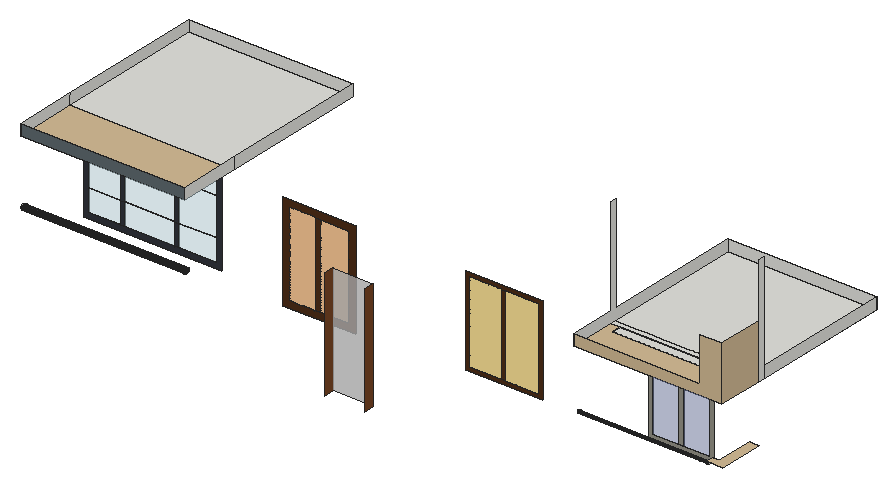
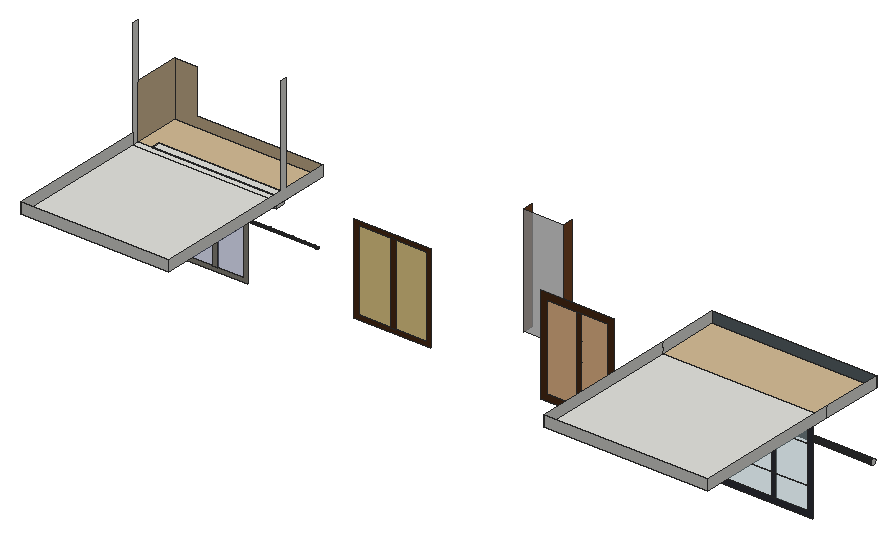
# SketchUp Ruby script. Lengths in inches.
U = 1.inch
M = Sketchup.active_model
def pt(a) = Geom::Point3d.new(a.map { |v| v * U })
def face(e, loops, mat)
  f = e.add_face(loops[0].map { |a| pt(a) })
  loops[1..].each { |l| e.add_face(l.map { |a| pt(a) }).erase! }
  f.material = f.back_material = mat if mat
  f
end
# faces: each face lists its corners as indices into pts; further lists are holes
def faces(e, pts, list, mat = nil) = list.each { |f| face(e, (f[0].is_a?(Array) ? f : [f]).map { |l| l.map { |i| pts[i] } }, mat) }
# xy, xz, yz: faces in a plane at the given z, y or x. An outline is a flat list of corners, or four numbers for a rectangle; further outlines are holes
def ring(l) = l.size == 4 ? [[l[0], l[1]], [l[2], l[1]], [l[2], l[3]], [l[0], l[3]]] : l.each_slice(2).to_a
def flat(e, list, mat, &to3) = list.each { |f| face(e, (f[0].is_a?(Array) ? f : [f]).map { |l| ring(l).map { |u, v| to3.(u, v) } }, mat) }
def xy(e, z, list, mat = nil) = flat(e, list, mat) { |x, y| [x, y, z] }
def xz(e, y, list, mat = nil) = flat(e, list, mat) { |x, z| [x, y, z] }
def yz(e, x, list, mat = nil) = flat(e, list, mat) { |y, z| [x, y, z] }
def lines(e, pts, list) = list.each { |a, b| e.add_line(pt(pts[a]), pt(pts[b])) }
# prism: a flat outline (further loops are holes) pulled along v
def prism(e, loops, v, mat = nil)
  f = face(e, loops, mat); d = Geom::Vector3d.new(v.map { |x| x * U })
  f.pushpull(f.normal.samedirection?(d) ? d.length : -d.length)
end
def box(e, o, s, mat = nil) = prism(e, [[o, [o[0] + s[0], o[1], o[2]], [o[0] + s[0], o[1] + s[1], o[2]], [o[0], o[1] + s[1], o[2]]]], [0, 0, s[2]], mat)
def at(x, y, z, deg = 0) = Geom::Transformation.translation(pt([x, y, z])) * Geom::Transformation.rotation(ORIGIN, Z_AXIS, deg.degrees)
def axes(o, x, y, z) = Geom::Transformation.new([*x, 0, *y, 0, *z, 0, *pt(o).to_a, 1])
def part(name) = M.definitions.add(name)
# library, detail: a bought-in or finely detailed component or shape, given as its bounding box
def library(name, o, s) = part(name).tap { |d| box(d.entities, o, s) }
def detail(e, o, s) = box(e.add_group.entities, o, s)
def put(e, d, t, mat = nil) = e.add_instance(d, t).tap { |i| i.material = mat if mat }
def group(e, t, mat = nil) = e.add_group.tap { |g| g.transformation = t; g.material = mat if mat }.entities
root = M.entities
M.materials.add("[Color C02]").color = [255, 204, 153]
M.materials.add("[Color D02]").color = [255, 229, 153]
M.materials.add("[Formica Beige]").color = [211, 187, 149]
M.materials.add("[Formica Graystone]").color = [149, 146, 135]
M.materials.add("[Formica Laminate Dark]").color = [50, 53, 60]
M.materials.add("[Formica Speckled Grey]").color = [94, 105, 111]
M.materials.add("[Translucent Glass Safety]").color = [204, 235, 244]
M.materials["[Translucent Glass Safety]"].alpha = 0.5
M.materials.add("[Translucent Glass Sky Reflection]").color = [126, 138, 183]
M.materials["[Translucent Glass Sky Reflection]"].alpha = 0.52
M.materials.add("[Translucent Resin Crush Gray]").color = [201, 201, 201]
M.materials["[Translucent Resin Crush Gray]"].alpha = 0.8
M.materials.add("[Wood Floor Light]").color = [204, 176, 127]
M.materials.add("[Wood Veneer 01]").color = [79, 46, 24]
M.materials.add("[Wood Veneer 01]2").color = [120, 70, 37]
xy(root,295.875,[[13.84,125.42,14.27,125.48,14.68,125.65,15.03,125.92,15.3,126.27,15.47,126.67,15.52,127.11,15.47,127.55,15.3,127.95,15.03,128.3,14.68,128.57,14.27,128.74,13.84,128.8,13.4,128.74,12.99,128.57,12.64,128.3,12.375,127.95,12.21,127.55,12.15,127.11,12.21,126.67,12.375,126.27,12.64,125.92,12.99,125.65,13.4,125.48]])
xy(root,296.125,[[101.27,125.42,101.71,125.48,102.12,125.65,102.47,125.92,102.74,126.27,102.9,126.67,102.96,127.11,102.9,127.55,102.74,127.95,102.47,128.3,102.12,128.57,101.71,128.74,101.27,128.8,100.84,128.74,100.43,128.57,100.08,128.3,99.8125,127.95,99.64,127.55,99.59,127.11,99.64,126.67,99.8125,126.27,100.08,125.92,100.43,125.65,100.84,125.48]])
xy(root,296.5,[[133.84,125.42,134.27,125.48,134.68,125.65,135.03,125.92,135.3,126.27,135.47,126.67,135.52,127.11,135.47,127.55,135.3,127.95,135.03,128.3,134.68,128.57,134.27,128.74,133.84,128.8,133.4,128.74,132.99,128.57,132.64,128.3,132.375,127.95,132.21,127.55,132.15,127.11,132.21,126.67,132.375,126.27,132.64,125.92,132.99,125.65,133.4,125.48]])
xy(root,296.625,[[118.77,125.42,119.21,125.48,119.62,125.65,119.97,125.92,120.24,126.27,120.4,126.67,120.46,127.11,120.4,127.55,120.24,127.95,119.97,128.3,119.62,128.57,119.21,128.74,118.77,128.8,118.34,128.74,117.93,128.57,117.58,128.3,117.3125,127.95,117.14,127.55,117.09,127.11,117.14,126.67,117.3125,126.27,117.58,125.92,117.93,125.65,118.34,125.48]])
xy(root,297.375,[[71.27,125.42,71.71,125.48,72.12,125.65,72.47,125.92,72.74,126.27,72.9,126.67,72.96,127.11,72.9,127.55,72.74,127.95,72.47,128.3,72.12,128.57,71.71,128.74,71.27,128.8,70.84,128.74,70.43,128.57,70.08,128.3,69.8125,127.95,69.64,127.55,69.59,127.11,69.64,126.67,69.8125,126.27,70.08,125.92,70.43,125.65,70.84,125.48]])
xy(root,297.49,[[42.4,125.42,42.84,125.48,43.24,125.65,43.59,125.92,43.86,126.27,44.03,126.67,44.09,127.11,44.03,127.55,43.86,127.95,43.59,128.3,43.24,128.57,42.84,128.74,42.4,128.8,41.96,128.74,41.56,128.57,41.21,128.3,40.9375,127.95,40.77,127.55,40.71,127.11,40.77,126.67,40.9375,126.27,41.21,125.92,41.56,125.65,41.96,125.48]])
xy(root,298.1875,[[27.09,125.42,27.52,125.48,27.93,125.65,28.28,125.92,28.55,126.27,28.72,126.67,28.77,127.11,28.72,127.55,28.55,127.95,28.28,128.3,27.93,128.57,27.52,128.74,27.09,128.8,26.65,128.74,26.24,128.57,25.89,128.3,25.625,127.95,25.46,127.55,25.4,127.11,25.46,126.67,25.625,126.27,25.89,125.92,26.24,125.65,26.65,125.48],[55.4,125.42,55.84,125.48,56.24,125.65,56.59,125.92,56.86,126.27,57.03,126.67,57.09,127.11,57.03,127.55,56.86,127.95,56.59,128.3,56.24,128.57,55.84,128.74,55.4,128.8,54.96,128.74,54.56,128.57,54.21,128.3,53.9375,127.95,53.77,127.55,53.71,127.11,53.77,126.67,53.9375,126.27,54.21,125.92,54.56,125.65,54.96,125.48],[149.84,125.42,150.27,125.48,150.68,125.65,151.03,125.92,151.3,126.27,151.47,126.67,151.52,127.11,151.47,127.55,151.3,127.95,151.03,128.3,150.68,128.57,150.27,128.74,149.84,128.8,149.4,128.74,148.99,128.57,148.64,128.3,148.375,127.95,148.21,127.55,148.15,127.11,148.21,126.67,148.375,126.27,148.64,125.92,148.99,125.65,149.4,125.48]])
xy(root,298.84,[[86.21,125.42,86.65,125.48,87.06,125.65,87.41,125.92,87.67,126.27,87.84,126.67,87.9,127.11,87.84,127.55,87.67,127.95,87.41,128.3,87.06,128.57,86.65,128.74,86.21,128.8,85.78,128.74,85.37,128.57,85.02,128.3,84.75,127.95,84.58,127.55,84.52,127.11,84.58,126.67,84.75,126.27,85.02,125.92,85.37,125.65,85.78,125.48],[167.96,125.42,168.4,125.48,168.81,125.65,169.16,125.92,169.42,126.27,169.59,126.67,169.65,127.11,169.59,127.55,169.42,127.95,169.16,128.3,168.81,128.57,168.4,128.74,167.96,128.8,167.53,128.74,167.12,128.57,166.77,128.3,166.5,127.95,166.33,127.55,166.27,127.11,166.33,126.67,166.5,126.27,166.77,125.92,167.12,125.65,167.53,125.48],[183.34,125.42,183.77,125.48,184.18,125.65,184.53,125.92,184.8,126.27,184.97,126.67,185.02,127.11,184.97,127.55,184.8,127.95,184.53,128.3,184.18,128.57,183.77,128.74,183.34,128.8,182.9,128.74,182.49,128.57,182.14,128.3,181.875,127.95,181.71,127.55,181.65,127.11,181.71,126.67,181.875,126.27,182.14,125.92,182.49,125.65,182.9,125.48]])
xy(root,301.75,[[674.41,135.92,674.75,135.96,675.07,136.09,675.34,136.3,675.55,136.57,675.68,136.89,675.72,137.23,675.68,137.57,675.55,137.88,675.34,138.16,675.07,138.36,674.75,138.5,674.41,138.54,674.07,138.5,673.75,138.36,673.48,138.16,673.27,137.88,673.14,137.57,673.1,137.23,673.14,136.89,673.27,136.57,673.48,136.3,673.75,136.09,674.07,135.96]],"[Formica Laminate Dark]")
xy(root,301.8125,[[628.3,136.16,628.61,136.2,628.9,136.32,629.14,136.51,629.33,136.76,629.45,137.04,629.49,137.35,629.45,137.66,629.33,137.94,629.14,138.19,628.9,138.38,628.61,138.5,628.3,138.54,627.99,138.5,627.71,138.38,627.46,138.19,627.27,137.94,627.16,137.66,627.11,137.35,627.16,137.04,627.27,136.76,627.46,136.51,627.71,136.32,627.99,136.2]],"[Formica Laminate Dark]")
xy(root,301.875,[[746.55,136.16,746.86,136.2,747.15,136.32,747.39,136.51,747.58,136.76,747.7,137.04,747.74,137.35,747.7,137.66,747.58,137.94,747.39,138.19,747.15,138.38,746.86,138.5,746.55,138.54,746.24,138.5,745.96,138.38,745.71,138.19,745.52,137.94,745.41,137.66,745.36,137.35,745.41,137.04,745.52,136.76,745.71,136.51,745.96,136.32,746.24,136.2]],"[Formica Laminate Dark]")
xy(root,301.91,[[651.47,136.9,653.64,136.9,653.7,137.04,653.74,137.35,653.7,137.66,653.58,137.94,653.39,138.19,653.15,138.38,652.86,138.5,652.55,138.54,652.24,138.5,651.96,138.38,651.71,138.19,651.52,137.94,651.41,137.66,651.36,137.35,651.41,137.04]])
xy(root,301.91,[[652.55,136.16,652.86,136.2,653.15,136.32,653.39,136.51,653.58,136.76,653.64,136.9,651.47,136.9,651.52,136.76,651.71,136.51,651.96,136.32,652.24,136.2]],"[Formica Laminate Dark]")
xy(root,301.9375,[[701.43,136.16,701.73,136.2,702.02,136.32,702.27,136.51,702.46,136.76,702.57,137.04,702.61,137.35,702.57,137.66,702.46,137.94,702.27,138.19,702.02,138.38,701.73,138.5,701.43,138.54,701.12,138.5,700.83,138.38,700.59,138.19,700.4,137.94,700.28,137.66,700.24,137.35,700.28,137.04,700.4,136.76,700.59,136.51,700.83,136.32,701.12,136.2]],"[Formica Laminate Dark]")
xy(root,302.125,[[684.99,136.16,685.3,136.2,685.58,136.32,685.83,136.51,686.02,136.76,686.14,137.04,686.18,137.35,686.14,137.66,686.02,137.94,685.83,138.19,685.58,138.38,685.3,138.5,684.99,138.54,684.68,138.5,684.4,138.38,684.15,138.19,683.96,137.94,683.84,137.66,683.8,137.35,683.84,137.04,683.96,136.76,684.15,136.51,684.4,136.32,684.68,136.2]],"[Formica Laminate Dark]")
xy(root,302.1875,[[735.74,136.16,736.05,136.2,736.33,136.32,736.58,136.51,736.77,136.76,736.89,137.04,736.93,137.35,736.89,137.66,736.77,137.94,736.58,138.19,736.33,138.38,736.05,138.5,735.74,138.54,735.43,138.5,735.15,138.38,734.9,138.19,734.71,137.94,734.59,137.66,734.55,137.35,734.59,137.04,734.71,136.76,734.9,136.51,735.15,136.32,735.43,136.2]],"[Formica Laminate Dark]")
xy(root,302.22,[[616.26,136.9375,618.47,136.9375,618.51,137.04,618.55,137.35,618.51,137.66,618.39,137.94,618.2,138.19,617.96,138.38,617.67,138.5,617.36,138.54,617.06,138.5,616.77,138.38,616.52,138.19,616.34,137.94,616.22,137.66,616.18,137.35,616.22,137.04]])
xy(root,302.22,[[617.36,136.16,617.67,136.2,617.96,136.32,618.2,136.51,618.39,136.76,618.47,136.9375,616.26,136.9375,616.34,136.76,616.52,136.51,616.77,136.32,617.06,136.2]],"[Formica Laminate Dark]")
xy(root,302.3125,[[640.36,136.16,640.67,136.2,640.96,136.32,641.2,136.51,641.39,136.76,641.51,137.04,641.55,137.35,641.51,137.66,641.39,137.94,641.2,138.19,640.96,138.38,640.67,138.5,640.36,138.54,640.06,138.5,639.77,138.38,639.52,138.19,639.34,137.94,639.22,137.66,639.18,137.35,639.22,137.04,639.34,136.76,639.52,136.51,639.77,136.32,640.06,136.2],[713.18,136.16,713.48,136.2,713.77,136.32,714.02,136.51,714.21,136.76,714.32,137.04,714.36,137.35,714.32,137.66,714.21,137.94,714.02,138.19,713.77,138.38,713.48,138.5,713.18,138.54,712.87,138.5,712.58,138.38,712.34,138.19,712.15,137.94,712.03,137.66,711.99,137.35,712.03,137.04,712.15,136.76,712.34,136.51,712.58,136.32,712.87,136.2]],"[Formica Laminate Dark]")
xy(root,302.375,[[724.8,136.16,725.11,136.2,725.4,136.32,725.64,136.51,725.83,136.76,725.95,137.04,725.99,137.35,725.95,137.66,725.83,137.94,725.64,138.19,725.4,138.38,725.11,138.5,724.8,138.54,724.49,138.5,724.21,138.38,723.96,138.19,723.77,137.94,723.66,137.66,723.61,137.35,723.66,137.04,723.77,136.76,723.96,136.51,724.21,136.32,724.49,136.2]],"[Formica Laminate Dark]")
xy(root,302.51,[[691.18,137.06,693.76,137.06,693.79,137.23,693.74,137.57,693.61,137.88,693.4,138.16,693.13,138.36,692.8125,138.5,692.47,138.54,692.13,138.5,691.82,138.36,691.55,138.16,691.34,137.88,691.21,137.57,691.16,137.23]])
xy(root,302.51,[[692.47,135.92,692.8125,135.96,693.13,136.09,693.4,136.3,693.61,136.57,693.74,136.89,693.76,137.06,691.18,137.06,691.21,136.89,691.34,136.57,691.55,136.3,691.82,136.09,692.13,135.96]],"[Formica Laminate Dark]")
xy(root,302.8125,[[665.36,136.16,665.67,136.2,665.96,136.32,666.2,136.51,666.39,136.76,666.51,137.04,666.55,137.35,666.51,137.66,666.39,137.94,666.2,138.19,665.96,138.38,665.67,138.5,665.36,138.54,665.06,138.5,664.77,138.38,664.52,138.19,664.34,137.94,664.22,137.66,664.18,137.35,664.22,137.04,664.34,136.76,664.52,136.51,664.77,136.32,665.06,136.2]],"[Formica Laminate Dark]")
xy(root,305.625,[[755.9375,133.3,774.15,133.3,774.15,182.57,764,182.57,764,141.82,755.9375,141.82]],"[Formica Beige]")
xy(root,356.625,[[621.3,172.64,641.63,182.57],[738.55,172.64,758.88,182.57]])
xy(root,356.625,[[641.63,172.64,738.55,182.57]],"[Wood Floor Light]")
xy(root,369,[[621.3,172.64,758.88,182.57],[621.3,172.64,758.88,182.57],[611.125,182.57,774.15,189.24],[611.125,189.24,774.15,344.36],[9,191.15,189.57,355.125]])
xy(root,369,[[9,122.79,189.57,191.15],[611.125,131.74,611.125,182.57,621.3,182.57,621.3,172.64,758.88,172.64,758.88,182.57,774.15,182.57,774.15,131.74]],"[Formica Beige]")
xz(root,88.2,[[380.3,262.65,424.94,384.08]],"[Translucent Resin Crush Gray]")
xz(root,122.79,[[9,369,189.57,381]],"[Formica Speckled Grey]")
xz(root,131.74,[[611.125,369,774.15,369,774.15,429,750.32,429,750.32,381,611.125,381]],"[Formica Beige]")
xz(root,172.64,[[621.3,356.625,758.88,369]],"[Wood Floor Light]")
xz(root,174.4375,[[264.12,273.03,292.18,365.2],[298.29,273.03,329.29,365.2]],"[Color C02]")
xz(root,174.4375,[[462.79,277.61,496.49,366.55],[502.51,277.61,537.84,366.55]],"[Color D02]")
xz(root,174.4375,[[[256.64,265.55,336.77,372.68],[264.12,273.03,329.29,365.2]],[292.18,273.03,298.29,365.2],[[458.21,273.03,542.42,371.125],[462.79,277.61,537.84,366.55]],[496.49,277.61,502.51,366.55]],"[Wood Veneer 01]")
xz(root,182.57,[[621.3,356.625,758.88,369]])
xz(root,182.57,[[[653.42,271.33,724.17,352.83],[657.48,275.39,720.12,348.77]],[685.82,275.39,691.11,348.77]],"[Formica Graystone]")
xz(root,182.57,[[657.48,275.39,685.82,348.77],[691.11,275.39,720.12,348.77]],"[Translucent Glass Sky Reflection]")
xz(root,191.15,[[[24.08,264.5,176.08,363],[29.79,270.2,170.375,357.29]],[64.72,270.2,69.58,294.48],[124.16,270.2,129.01,294.48],[64.72,294.48,69.58,336.17],[124.16,294.48,129.01,336.17],
  [64.72,336.17,69.58,357.29],[124.16,336.17,129.01,357.29]],"[Formica Laminate Dark]")
xz(root,191.15,[[29.79,270.2,64.72,294.48],[69.58,270.2,124.16,294.48],[129.01,270.2,170.375,294.48],[29.79,294.48,64.72,336.17],[69.58,294.48,124.16,336.17],
  [129.01,294.48,170.375,336.17],[29.79,336.17,64.72,357.29],[69.58,336.17,124.16,357.29],[129.01,336.17,170.375,357.29]],"[Translucent Glass Safety]")
xz(root,344.36,[[611.125,369,774.15,381]])
xz(root,355.125,[[9,369,189.57,381]])
yz(root,9,[[126.49,294.81,125.8,294.9,125.15,295.17,124.59,295.59,124.17,296.15,123.9,296.8,123.81,297.49,123.9,298.1875,124.17,298.84,124.59,299.39,125.15,299.82,125.8,300.09,126.49,300.18,127.1875,300.09,127.84,299.82,128.39,299.39,128.82,298.84,129.09,298.1875,129.18,297.49,129.09,296.8,128.82,296.15,128.39,295.59,127.84,295.17,127.1875,294.9],[122.79,369,191.15,381],[191.15,369,355.125,381]])
yz(root,189.57,[[122.79,369,191.15,381],[191.15,369,355.125,381]])
yz(root,380.3,[[77.26,262.65,88.2,384.08]],"[Wood Veneer 01]2")
yz(root,424.94,[[77.26,262.65,88.2,384.08]],"[Wood Veneer 01]2")
yz(root,611.125,[[131.74,369,344.36,369,344.36,381,189.24,381,189.24,489,182.57,489,182.57,381,131.74,381]])
yz(root,621.3,[[172.64,356.625,182.57,369]])
yz(root,755.9375,[[138.08,300.72,138.39,300.77,138.68,300.88,138.92,301.07,139.11,301.32,139.23,301.6,139.27,301.91,139.23,302.22,139.11,302.51,138.92,302.75,138.68,302.94,138.39,303.06,138.08,303.1,137.78,303.06,137.49,302.94,137.25,302.75,137.06,302.51,136.9375,302.22,136.9,301.91,136.9375,301.6,137.06,301.32,137.25,301.07,137.49,300.88,137.78,300.77]])
yz(root,758.88,[[172.64,356.625,182.57,369]],"[Formica Beige]")
yz(root,774.15,[[182.57,369,189.24,489],[189.24,369,344.36,381]])
yz(root,774.15,[[131.74,369,182.57,429]],"[Formica Beige]")
p = [[9,125.8,294.9],[9,126.49,294.81],[189.57,126.49,294.81],[189.57,125.8,294.9],[9,127.1875,294.9],[189.57,127.1875,294.9],
  [9,125.15,295.17],[189.57,125.15,295.17],[9,127.84,295.17],[189.57,127.84,295.17],[9,124.59,295.59],[189.57,124.59,295.59],
  [9,128.39,295.59],[189.57,128.39,295.59],[9,124.17,296.15],[189.57,124.17,296.15],[9,128.82,296.15],[189.57,128.82,296.15],
  [9,123.9,296.8],[189.57,123.9,296.8],[9,129.09,296.8],[189.57,129.09,296.8],[9,123.81,297.49],[189.57,123.81,297.49],
  [9,129.18,297.49],[189.57,129.18,297.49],[9,123.9,298.1875],[189.57,123.9,298.1875],[9,129.09,298.1875],[189.57,129.09,298.1875],
  [9,124.17,298.84],[189.57,124.17,298.84],[9,128.82,298.84],[189.57,128.82,298.84],[9,124.59,299.39],[189.57,124.59,299.39],
  [9,128.39,299.39],[189.57,128.39,299.39],[9,125.15,299.82],[189.57,125.15,299.82],[9,127.84,299.82],[189.57,127.84,299.82],
  [9,125.8,300.09],[189.57,125.8,300.09],[9,127.1875,300.09],[189.57,127.1875,300.09],[9,126.49,300.18],[189.57,126.49,300.18],
  [755.9375,138.08,300.72],[755.9375,137.78,300.77],[611.125,137.78,300.77],[611.125,138.08,300.72],[755.9375,138.39,300.77],[611.125,138.39,300.77],
  [755.9375,137.49,300.88],[611.125,137.49,300.88],[755.9375,138.68,300.88],[611.125,138.68,300.88],[755.9375,137.25,301.07],[611.125,137.25,301.07],
  [755.9375,138.92,301.07],[611.125,138.92,301.07],[755.9375,137.06,301.32],[611.125,137.06,301.32],[755.9375,139.11,301.32],[611.125,139.11,301.32],
  [755.9375,136.9375,301.6],[611.125,136.9375,301.6],[755.9375,139.23,301.6],[611.125,139.23,301.6],[755.9375,136.9,301.91],[653.64,136.9,301.91],
  [651.47,136.9,301.91],[611.125,136.9,301.91],[755.9375,139.27,301.91],[611.125,139.27,301.91],[755.9375,136.9375,302.22],[618.47,136.9375,302.22],
  [616.26,136.9375,302.22],[611.125,136.9375,302.22],[755.9375,139.23,302.22],[611.125,139.23,302.22],[755.9375,137.06,302.51],[693.76,137.06,302.51],
  [691.18,137.06,302.51],[611.125,137.06,302.51],[755.9375,139.11,302.51],[611.125,139.11,302.51],[755.9375,137.25,302.75],[611.125,137.25,302.75],
  [755.9375,138.92,302.75],[611.125,138.92,302.75],[755.9375,137.49,302.94],[611.125,137.49,302.94],[755.9375,138.68,302.94],[611.125,138.68,302.94],
  [755.9375,137.78,303.06],[611.125,137.78,303.06],[755.9375,138.39,303.06],[611.125,138.39,303.06],[755.9375,138.08,303.1],[611.125,138.08,303.1]]
faces(root,p,[[0,1,2,3],[1,4,5,2],[6,0,3,7],[4,8,9,5],[10,6,7,11],[8,12,13,9],[14,10,11,15],[12,16,17,13],
  [18,14,15,19],[16,20,21,17],[22,18,19,23],[20,24,25,21],[26,22,23,27],[24,28,29,25],[30,26,27,31],[28,32,33,29],
  [34,30,31,35],[32,36,37,33],[38,34,35,39],[36,40,41,37],[42,38,39,43],[40,44,45,41],[46,42,43,47],[44,46,47,45],
  [48,49,50,51],[52,48,51,53],[49,54,55,50],[56,52,53,57],[54,58,59,55],[60,56,57,61],[58,62,63,59],[64,60,61,65],
  [62,66,67,63],[68,64,65,69],[66,70,71,72,73,67],[74,68,69,75],[70,76,77,78,79,73,72,71],[80,74,75,81],[76,82,83,84,85,79,78,77],[86,80,81,87],
  [82,88,89,85,84,83],[90,86,87,91],[88,92,93,89],[94,90,91,95],[92,96,97,93],[98,94,95,99],[96,100,101,97],[100,98,99,101]],"[Formica Laminate Dark]")
